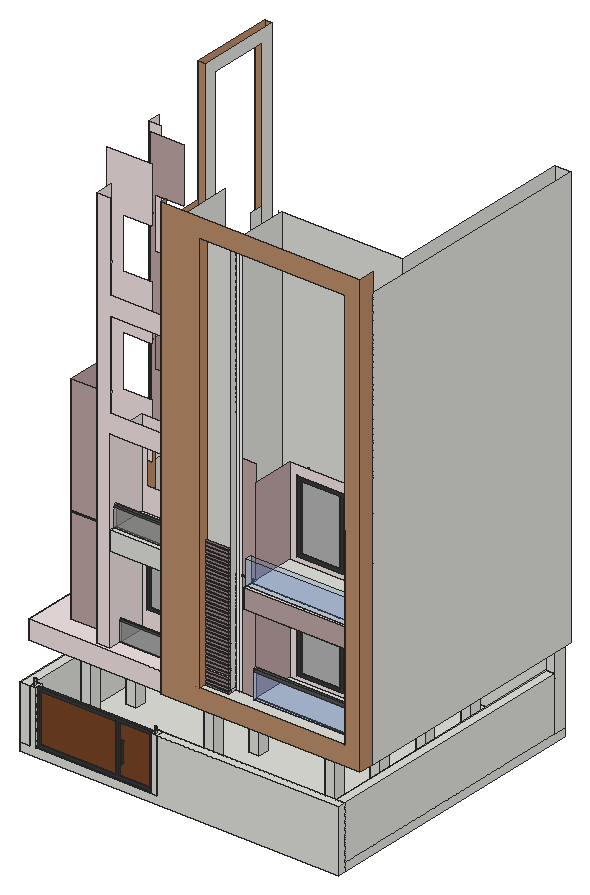
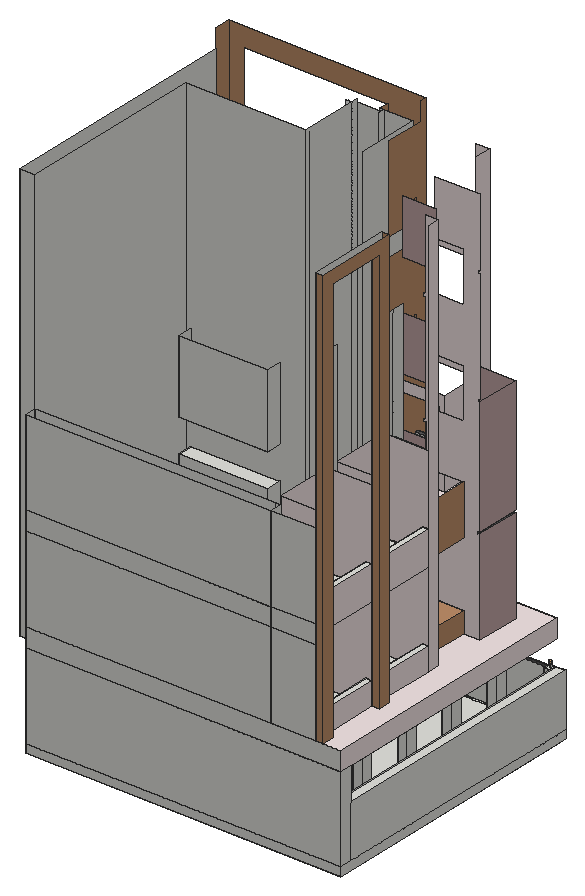
# SketchUp Ruby script. Lengths in inches.
U = 1.inch
M = Sketchup.active_model
def pt(a) = Geom::Point3d.new(a.map { |v| v * U })
def face(e, loops, mat)
  f = e.add_face(loops[0].map { |a| pt(a) })
  loops[1..].each { |l| e.add_face(l.map { |a| pt(a) }).erase! }
  f.material = f.back_material = mat if mat
  f
end
# faces: each face lists its corners as indices into pts; further lists are holes
def faces(e, pts, list, mat = nil) = list.each { |f| face(e, (f[0].is_a?(Array) ? f : [f]).map { |l| l.map { |i| pts[i] } }, mat) }
# xy, xz, yz: faces in a plane at the given z, y or x. An outline is a flat list of corners, or four numbers for a rectangle; further outlines are holes
def ring(l) = l.size == 4 ? [[l[0], l[1]], [l[2], l[1]], [l[2], l[3]], [l[0], l[3]]] : l.each_slice(2).to_a
def flat(e, list, mat, &to3) = list.each { |f| face(e, (f[0].is_a?(Array) ? f : [f]).map { |l| ring(l).map { |u, v| to3.(u, v) } }, mat) }
def xy(e, z, list, mat = nil) = flat(e, list, mat) { |x, y| [x, y, z] }
def xz(e, y, list, mat = nil) = flat(e, list, mat) { |x, z| [x, y, z] }
def yz(e, x, list, mat = nil) = flat(e, list, mat) { |y, z| [x, y, z] }
def lines(e, pts, list) = list.each { |a, b| e.add_line(pt(pts[a]), pt(pts[b])) }
# prism: a flat outline (further loops are holes) pulled along v
def prism(e, loops, v, mat = nil)
  f = face(e, loops, mat); d = Geom::Vector3d.new(v.map { |x| x * U })
  f.pushpull(f.normal.samedirection?(d) ? d.length : -d.length)
end
def box(e, o, s, mat = nil) = prism(e, [[o, [o[0] + s[0], o[1], o[2]], [o[0] + s[0], o[1] + s[1], o[2]], [o[0], o[1] + s[1], o[2]]]], [0, 0, s[2]], mat)
def at(x, y, z, deg = 0) = Geom::Transformation.translation(pt([x, y, z])) * Geom::Transformation.rotation(ORIGIN, Z_AXIS, deg.degrees)
def axes(o, x, y, z) = Geom::Transformation.new([*x, 0, *y, 0, *z, 0, *pt(o).to_a, 1])
def part(name) = M.definitions.add(name)
# library, detail: a bought-in or finely detailed component or shape, given as its bounding box
def library(name, o, s) = part(name).tap { |d| box(d.entities, o, s) }
def detail(e, o, s) = box(e.add_group.entities, o, s)
def put(e, d, t, mat = nil) = e.add_instance(d, t).tap { |i| i.material = mat if mat }
def group(e, t, mat = nil) = e.add_group.tap { |g| g.transformation = t; g.material = mat if mat }.entities
root = M.entities
M.materials.add("Generic\#1").color = [192, 166, 166]
M.materials.add("Generic\#2").color = [190, 142, 105]
M.materials.add("Generic\#3").color = [158, 131, 131]
M.materials.add("Generic\#4").color = [242, 228, 228]
M.materials.add("[Color M00]").color = [255, 255, 255]
M.materials.add("[Color M06]").color = [86, 86, 86]
M.materials.add("[Color M07]").color = [58, 58, 58]
M.materials.add("[Mirror 01]").color = [183, 183, 183]
M.materials.add("[Translucent Glass Blue]").color = [98, 147, 234]
M.materials["[Translucent Glass Blue]"].alpha = 0.21
M.materials.add("[Translucent Glass Gray]").color = [128, 128, 128]
M.materials["[Translucent Glass Gray]"].alpha = 0.5
M.materials.add("[Wood Veneer 01]").color = [120, 70, 37]
c1 = part("Group\#3")
xy(c1.entities,0,[[0,0,45.875,5.125]])
xz(c1.entities,0,[[0,0,45.875,4.1875]])
yz(c1.entities,45.875,[[0,0,5.125,4.1875]])
c2 = part("Group\#2")
xy(c2.entities,0,[[0,0,173,6]],"[Color M07]")
xy(c2.entities,7.67,[[90.33,0,165.33,3]],"[Color M06]")
xy(c2.entities,7.67,[[7.67,0,82.67,3]],"[Color M07]")
xy(c2.entities,134.58,[[7.67,0,82.67,3],[90.33,0,165.33,3]],"[Color M07]")
xy(c2.entities,142.25,[[0,0,173,6]],"[Color M07]")
xz(c2.entities,0,[[[0,0,173,142.25],[7.67,7.67,82.67,134.58],[90.33,7.67,165.33,134.58]]],"[Color M07]")
xz(c2.entities,3,[[7.67,7.67,82.67,134.58],[90.33,7.67,165.33,134.58]],"[Mirror 01]")
xz(c2.entities,6,[[0,0,173,142.25]],"[Mirror 01]")
yz(c2.entities,0,[[0,0,6,142.25]],"[Color M07]")
yz(c2.entities,7.67,[[0,7.67,3,134.58]],"[Color M07]")
yz(c2.entities,82.67,[[0,7.67,3,134.58]],"[Color M07]")
yz(c2.entities,90.33,[[0,7.67,3,134.58]],"[Color M07]")
yz(c2.entities,165.33,[[0,7.67,3,134.58]],"[Color M07]")
yz(c2.entities,173,[[0,0,6,142.25]],"[Color M07]")
c3 = part("Group\#1")
xy(c3.entities,0,[[0,0,90.75,6]],"[Color M07]")
xy(c3.entities,5.41,[[5.41,0,42.67,3],[48.08,0,85.34,3]],"[Color M07]")
xy(c3.entities,95.34,[[5.41,0,42.67,3],[48.08,0,85.34,3]],"[Color M07]")
xy(c3.entities,100.75,[[0,0,90.75,6]],"[Color M07]")
xz(c3.entities,0,[[[0,0,90.75,100.75],[48.08,5.41,85.34,95.34],[5.41,5.41,42.67,95.34]]],"[Color M07]")
xz(c3.entities,3,[[5.41,5.41,42.67,95.34],[48.08,5.41,85.34,95.34]],"[Mirror 01]")
xz(c3.entities,6,[[0,0,90.75,100.75]],"[Mirror 01]")
yz(c3.entities,0,[[0,0,6,100.75]],"[Color M07]")
yz(c3.entities,5.41,[[0,5.41,3,95.34]],"[Color M07]")
yz(c3.entities,42.67,[[0,5.41,3,95.34]],"[Color M07]")
yz(c3.entities,48.08,[[0,5.41,3,95.34]],"[Color M07]")
yz(c3.entities,85.34,[[0,5.41,3,95.34]],"[Color M07]")
yz(c3.entities,90.75,[[0,0,6,100.75]],"[Color M07]")
xy(root,-15.875,[[0,0,617.3125,15.0625],[0,15.0625,617.3125,549.6875]])
xy(root,0,[[0,0,18.4375,15.0625],[30.125,0,253,15.0625],[253,0,264.6875,15.0625],[0,15.0625,18.4375,525.6875],[[18.4375,15.0625,599.75,525.6875],[52.22,82.12,71.54,103.62],[52.22,191.41,71.54,212.91],[52.22,300.71,71.54,322.21],[52.22,410,71.54,431.5],[290.41,410,309.72,431.5],[290.41,300.71,309.72,322.21],[290.41,191.41,309.72,212.91],[290.41,82.12,309.72,103.62],[526.0625,410,545.375,431.5],[526.0625,300.71,545.375,322.21],[526.0625,191.41,545.375,212.91],[526.0625,82.12,545.375,103.62]],
  [599.75,15.0625,617.3125,525.6875],[52.22,82.12,71.54,103.62],[290.41,82.12,309.72,103.62],[526.0625,82.12,545.375,103.62],[52.22,191.41,71.54,212.91],
  [290.41,191.41,309.72,212.91],[526.0625,191.41,545.375,212.91],[52.22,300.71,71.54,322.21],[290.41,300.71,309.72,322.21],[526.0625,300.71,545.375,322.21],
  [52.22,410,71.54,431.5],[290.41,410,309.72,431.5],[526.0625,410,545.375,431.5],[0,525.6875,617.3125,549.6875]])
xy(root,104.18,[[0,0,18.4375,525.6875],[[18.4375,0,30.125,15.0625],[23.27,4.73,25.7,7.24]],[[253,0,264.6875,15.0625],[257.17,4.73,259.61,7.24]],[264.6875,0,617.3125,15.0625],[23.27,4.73,25.7,7.24],
  [257.17,4.73,259.61,7.24],[599.75,15.0625,617.3125,525.6875]])
xy(root,110.18,[[23.27,4.73,25.7,7.24],[257.17,4.73,259.61,7.24]])
xy(root,168,[[[261.3125,15.0625,261.3125,20.375,0,20.375,0,525.6875,647.125,525.6875,647.125,15.0625],[52.22,82.12,71.54,103.62],[52.22,191.41,71.54,212.91],[52.22,300.71,71.54,322.21],[52.22,410,71.54,431.5],[526.0625,82.12,545.375,103.62],[526.0625,191.41,545.375,212.91],[526.0625,300.71,545.375,322.21],[526.0625,410,545.375,431.5],[290.41,410,309.72,431.5],[290.41,300.71,309.72,322.21],[290.41,191.41,309.72,212.91],[290.41,82.12,309.72,103.62]],[0,525.6875,617.3125,549.6875]])
xy(root,204.5625,[[336,15.0625,617.3125,15.0625,617.3125,39,421.3125,39,421.3125,45.6875,381.875,45.6875,381.875,33.8125,336,33.8125],[271.74,33.8125,271.74,157.1,137.3125,157.1,137.3125,525.6875,617.3125,525.6875,617.3125,157.1,381.875,157.1,381.875,45.6875,328.375,45.6875,328.375,33.8125],[328.375,33.8125,381.875,45.6875],[421.3125,45.6875,617.3125,128.4375],[152.75,50.125,261.3125,53.5625],
  [80.75,147.9375,137.3125,225.85],[73.1875,225.85,137.3125,249.85],[49.25,249.85,137.3125,273.85],[61.25,273.85,137.3125,387.77],[34.875,387.77,49.25,411.77],
  [49.25,387.77,137.3125,411.77],[61.25,411.77,137.3125,525.6875],[34.875,525.6875,49.25,549.6875],[49.25,525.6875,137.3125,549.6875],[137.3125,525.6875,617.3125,549.6875]])
xy(root,204.5625,[[0,20.375,261.3125,20.375,261.3125,50.125,152.75,50.125,152.75,27.5625,126.1875,27.5625,126.1875,61.3125,49.25,61.3125,49.25,147.9375,80.75,147.9375,80.75,225.85,73.1875,225.85,73.1875,249.85,49.25,249.85,49.25,387.77,34.875,387.77,34.875,411.77,49.25,411.77,49.25,525.6875,34.875,525.6875,34.875,549.6875,0,549.6875]],"Generic\#4")
xy(root,204.5625,[[152.75,53.5625,261.3125,105]],"[Color M00]")
xy(root,209.0625,[[375.18,33.8125,381.875,157.1]])
xy(root,209.87,[[434.09,128.4375,607.09,187.0625]])
xy(root,240.21,[[162.625,105,253.375,171.75]])
xy(root,241.5,[[152.75,50.125,261.3125,53.5625]])
xy(root,245.0625,[[152.75,50.125,261.3125,53.5625]],"[Color M06]")
xy(root,245.625,[[80.75,147.9375,137.3125,225.85]],"Generic\#2")
xy(root,249.6875,[[49.25,273.85,61.25,387.77],[49.25,411.77,61.25,525.6875]])
xy(root,252.5625,[[421.3125,39,617.3125,45.6875]])
xy(root,258,[[421.3125,39,617.3125,45.6875]],"[Color M06]")
xy(root,340.96,[[162.625,105,253.375,171.75]])
xy(root,352.12,[[434.09,128.4375,607.09,187.0625]])
xy(root,372.5625,[[137.3125,525.6875,617.3125,549.6875]])
xy(root,372.5625,[[421.3125,15.0625,617.3125,128.4375],[80.75,147.9375,137.3125,225.85]],"Generic\#2")
xy(root,372.5625,[[152.75,27.5625,261.3125,105]],"Generic\#4")
xy(root,378.72,[[73.1875,225.85,77.875,249.85]],"[Color M06]")
xy(root,384.87,[[73.1875,225.85,77.875,249.85]],"[Color M06]")
xy(root,387.625,[[49.25,273.85,137.3125,387.77],[49.25,411.77,137.3125,525.6875]],"Generic\#4")
xy(root,390.07,[[49.25,61.3125,126.1875,66],[49.25,66,53.9375,147.9375]],"[Color M06]")
xy(root,394.07,[[49.25,61.3125,126.1875,66],[49.25,66,53.9375,147.9375]],"[Color M06]")
xy(root,406.125,[[392.6875,45.6875,421.3125,49.375]])
xy(root,409.125,[[421.3125,15.0625,617.3125,20.9],[421.3125,20.9,617.3125,32.9],[152.75,27.5625,261.3125,35.875],[421.3125,32.9,617.3125,128.4375],[152.75,35.875,261.3125,42.5625],
  [152.75,42.5625,261.3125,105],[392.6875,45.6875,421.3125,49.375],[61.25,273.85,137.3125,387.77],[61.25,411.77,137.3125,525.6875],[137.3125,525.6875,617.3125,549.6875]])
xy(root,417.43,[[434.09,128.4375,607.09,187.0625]])
xy(root,446.0625,[[152.75,35.875,261.3125,42.5625]])
xy(root,449.625,[[152.75,35.875,261.3125,42.5625]],"[Color M06]")
xy(root,454.25,[[49.25,273.85,61.25,387.77],[49.25,411.77,61.25,525.6875]])
xz(root,0,[[0,-15.875,617.3125,-15.875,617.3125,104.18,264.6875,104.18,264.6875,0,30.125,0,30.125,104.18,18.4375,104.18,18.4375,0,0,0],[0,0,18.4375,104.18],[253,0,264.6875,104.18]])
xz(root,4.73,[[23.27,104.18,25.7,110.18],[257.17,104.18,259.61,110.18]])
xz(root,7.24,[[23.27,104.18,25.7,110.18],[257.17,104.18,259.61,110.18]])
xz(root,15.0625,[[18.4375,0,30.125,104.18],[253,0,264.6875,104.18],[264.6875,0,599.75,104.18],[599.75,0,617.3125,104.18]])
xz(root,15.0625,[[421.3125,372.5625,617.3125,409.125]],"Generic\#1")
xz(root,15.0625,[[[261.3125,168,647.125,1022.8125],[336,204.5625,617.3125,986.25]]],"Generic\#2")
xz(root,20.375,[[0,168,261.3125,204.5625]],"Generic\#4")
xz(root,20.9,[[421.3125,409.125,617.3125,457.125]],"[Translucent Glass Blue]")
xz(root,27.5625,[[152.75,372.5625,261.3125,409.125]])
xz(root,27.5625,[[126.1875,204.5625,152.75,204.5625,152.75,577.125,261.3125,577.125,261.3125,613.6875,152.75,613.6875,152.75,781.6875,261.3125,781.6875,261.3125,818.25,152.75,818.25,152.75,986.25,126.1875,986.25]],"Generic\#4")
xz(root,32.9,[[421.3125,409.125,617.3125,457.125]],"[Translucent Glass Blue]")
xz(root,33.8125,[[271.74,204.5625,328.375,986.25],[328.375,204.5625,336,986.25],[336,204.5625,381.875,982.0625]])
xz(root,35.875,[[152.75,446.0625,261.3125,449.625]],"[Color M06]")
xz(root,35.875,[[152.75,409.125,261.3125,446.0625]],"[Translucent Glass Gray]")
xz(root,39,[[421.3125,252.5625,617.3125,258]],"[Color M06]")
xz(root,39,[[421.3125,204.5625,617.3125,252.5625]],"[Translucent Glass Blue]")
xz(root,42.5625,[[152.75,446.0625,261.3125,449.625]])
xz(root,42.5625,[[152.75,409.125,261.3125,446.0625]],"[Translucent Glass Gray]")
xz(root,45.6875,[[421.3125,252.5625,617.3125,258]])
xz(root,45.6875,[[392.6875,204.5625,421.3125,406.125],[392.6875,409.125,421.3125,610.6875]],"Generic\#1")
xz(root,45.6875,[[381.875,204.5625,392.6875,986.25]],"[Color M00]")
xz(root,45.6875,[[421.3125,204.5625,617.3125,252.5625]],"[Translucent Glass Blue]")
xz(root,49.375,[[392.6875,406.125,421.3125,409.125]],"[Color M06]")
xz(root,50.125,[[152.75,241.5,261.3125,245.0625]],"[Color M06]")
xz(root,50.125,[[152.75,204.5625,261.3125,241.5]],"[Translucent Glass Gray]")
xz(root,53.5625,[[152.75,241.5,261.3125,245.0625]])
xz(root,53.5625,[[152.75,204.5625,261.3125,241.5]],"[Translucent Glass Gray]")
xz(root,61.3125,[[49.25,204.5625,126.1875,390.07],[49.25,394.07,126.1875,621.63]],"Generic\#1")
xz(root,66,[[53.9375,390.07,126.1875,394.07]],"[Color M06]")
xz(root,82.12,[[52.22,0,71.54,168],[290.41,0,309.72,168],[526.0625,0,545.375,168]])
xz(root,103.62,[[52.22,0,71.54,168],[290.41,0,309.72,168],[526.0625,0,545.375,168]])
xz(root,105,[[[152.75,204.5625,261.3125,372.5625],[162.625,240.21,253.375,340.96]],[[152.75,409.125,261.3125,577.125],[162.5,455.21,253.25,555.96]]],"Generic\#4")
xz(root,128.4375,[[[421.3125,204.5625,617.3125,372.5625],[434.09,209.87,607.09,352.12]],[[421.3125,409.125,617.3125,577.125],[434.09,417.43,607.09,559.68]]],"Generic\#4")
xz(root,147.9375,[[80.75,204.5625,137.3125,245.625]])
xz(root,147.9375,[[49.25,204.5625,49.25,390.07,53.9375,390.07,53.9375,394.07,49.25,394.07,49.25,621.63,53.9375,621.63,53.9375,625.63,49.25,625.63,49.25,847.32,53.9375,847.32,53.9375,851.32,49.25,851.32,49.25,986.25,137.3125,986.25,137.3125,879.375,80.75,879.375,80.75,781.6875,137.3125,781.6875,137.3125,674.8125,80.75,674.8125,80.75,577.125,137.3125,577.125,137.3125,470.25,80.75,470.25,80.75,372.5625,137.3125,372.5625,137.3125,245.625,80.75,245.625,80.75,204.5625]],"Generic\#4")
xz(root,157.1,[[381.875,204.5625,617.3125,986.25]])
xz(root,171.75,[[162.625,240.21,253.375,340.96]])
xz(root,187.0625,[[434.09,209.87,607.09,352.12],[434.09,417.43,607.09,559.68]])
xz(root,191.41,[[52.22,0,71.54,168],[290.41,0,309.72,168],[526.0625,0,545.375,168]])
xz(root,212.91,[[52.22,0,71.54,168],[290.41,0,309.72,168],[526.0625,0,545.375,168]])
xz(root,225.85,[[80.75,204.5625,137.3125,245.625],[80.75,372.5625,137.3125,470.25]])
xz(root,225.85,[[73.1875,204.5625,80.75,204.5625,80.75,245.625,137.3125,245.625,137.3125,372.5625,80.75,372.5625,80.75,470.25,137.3125,470.25,137.3125,577.125,80.75,577.125,80.75,674.8125,137.3125,674.8125,137.3125,781.6875,80.75,781.6875,80.75,879.375,137.3125,879.375,137.3125,986.25,73.1875,986.25,73.1875,847.44,77.875,847.44,77.875,843.44,73.1875,843.44,73.1875,627.77,77.875,627.77,77.875,623.77,73.1875,623.77,73.1875,384.87,77.875,384.87,77.875,378.72,73.1875,378.72]],"Generic\#1")
xz(root,249.85,[[73.1875,204.5625,137.3125,372.5625],[73.1875,372.5625,137.3125,372.5625,137.3125,409.125,73.1875,409.125,73.1875,384.87,77.875,384.87,77.875,378.72,73.1875,378.72],[73.1875,409.125,137.3125,577.125]])
xz(root,249.85,[[49.25,204.5625,73.1875,204.5625,73.1875,378.72,77.875,378.72,77.875,384.87,73.1875,384.87,73.1875,623.77,77.875,623.77,77.875,627.77,73.1875,627.77,73.1875,843.44,77.875,843.44,77.875,847.44,73.1875,847.44,73.1875,986.25,49.25,986.25]],"Generic\#4")
xz(root,273.85,[[49.25,204.5625,61.25,249.6875],[49.25,387.625,49.25,454.25,61.25,454.25,61.25,409.125,137.3125,409.125,137.3125,387.625]])
xz(root,273.85,[[61.25,204.5625,61.25,249.6875,49.25,249.6875,49.25,387.625,137.3125,387.625,137.3125,204.5625],[61.25,409.125,61.25,454.25,49.25,454.25,49.25,592.1875,137.3125,592.1875,137.3125,409.125]],"Generic\#4")
xz(root,300.71,[[52.22,0,71.54,168],[290.41,0,309.72,168],[526.0625,0,545.375,168]])
xz(root,322.21,[[52.22,0,71.54,168],[290.41,0,309.72,168],[526.0625,0,545.375,168]])
xz(root,387.77,[[49.25,204.5625,61.25,249.6875],[49.25,387.625,137.3125,387.625,137.3125,409.125,61.25,409.125,61.25,454.25,49.25,454.25]])
xz(root,387.77,[[34.875,204.5625,49.25,1024.8125]],"Generic\#2")
xz(root,387.77,[[61.25,204.5625,137.3125,204.5625,137.3125,387.625,49.25,387.625,49.25,249.6875,61.25,249.6875],[61.25,409.125,137.3125,409.125,137.3125,592.1875,49.25,592.1875,49.25,454.25,61.25,454.25]],"Generic\#4")
xz(root,410,[[52.22,0,71.54,168],[290.41,0,309.72,168],[526.0625,0,545.375,168]])
xz(root,411.77,[[49.25,204.5625,61.25,249.6875],[49.25,387.625,49.25,454.25,61.25,454.25,61.25,409.125,137.3125,409.125,137.3125,387.625]])
xz(root,411.77,[[34.875,204.5625,49.25,1000.9375]],"Generic\#2")
xz(root,411.77,[[61.25,204.5625,61.25,249.6875,49.25,249.6875,49.25,387.625,137.3125,387.625,137.3125,204.5625],[61.25,409.125,61.25,454.25,49.25,454.25,49.25,592.1875,137.3125,592.1875,137.3125,409.125]],"Generic\#4")
xz(root,431.5,[[52.22,0,71.54,168],[290.41,0,309.72,168],[526.0625,0,545.375,168]])
xz(root,525.6875,[[0,0,18.4375,104.18],[18.4375,0,599.75,168],[599.75,0,617.3125,104.18],[0,104.18,18.4375,168],[599.75,104.18,617.3125,168],
  [617.3125,168,647.125,986.25],[49.25,204.5625,61.25,249.6875],[137.3125,204.5625,145.6875,372.5625],[145.6875,204.5625,617.3125,372.5625],[137.3125,372.5625,145.6875,409.125],
  [145.6875,372.5625,617.3125,409.125],[49.25,387.625,137.3125,387.625,137.3125,409.125,61.25,409.125,61.25,454.25,49.25,454.25],[137.3125,409.125,145.6875,577.125],[145.6875,409.125,617.3125,577.125]])
xz(root,525.6875,[[34.875,204.5625,49.25,1000.9375]],"Generic\#2")
xz(root,525.6875,[[61.25,204.5625,137.3125,204.5625,137.3125,387.625,49.25,387.625,49.25,249.6875,61.25,249.6875],[61.25,409.125,137.3125,409.125,137.3125,592.1875,49.25,592.1875,49.25,454.25,61.25,454.25]],"Generic\#4")
xz(root,549.6875,[[0,-15.875,617.3125,0],[0,0,617.3125,168],[0,168,617.3125,204.5625],[49.25,204.5625,137.3125,372.5625],[137.3125,204.5625,617.3125,372.5625],
  [49.25,372.5625,137.3125,409.125],[137.3125,372.5625,617.3125,409.125],[49.25,409.125,137.3125,577.125],[137.3125,409.125,617.3125,577.125]])
xz(root,549.6875,[[34.875,204.5625,49.25,1024.8125]],"Generic\#2")
yz(root,0,[[0,-15.875,549.6875,0],[0,0,525.6875,104.18],[525.6875,0,549.6875,168]])
yz(root,0,[[20.375,168,549.6875,204.5625]],"Generic\#4")
yz(root,18.4375,[[0,0,15.0625,104.18],[15.0625,0,525.6875,104.18]])
yz(root,23.27,[[4.73,104.18,7.24,110.18]])
yz(root,25.7,[[4.73,104.18,7.24,110.18]])
yz(root,30.125,[[0,0,15.0625,104.18]])
yz(root,34.875,[[387.77,204.5625,387.77,1024.8125,549.6875,1024.8125,549.6875,204.5625,525.6875,204.5625,525.6875,1000.9375,411.77,1000.9375,411.77,204.5625]],"Generic\#2")
yz(root,49.25,[[387.77,204.5625,411.77,204.5625,411.77,1000.9375,525.6875,1000.9375,525.6875,204.5625,549.6875,204.5625,549.6875,1024.8125,387.77,1024.8125]])
yz(root,49.25,[[61.3125,204.5625,147.9375,390.07],[61.3125,394.07,147.9375,621.63]],"Generic\#1")
yz(root,49.25,[[249.85,204.5625,273.85,986.25],[273.85,204.5625,387.77,249.6875],[411.77,204.5625,525.6875,249.6875],[273.85,387.625,387.77,454.25],[411.77,387.625,525.6875,454.25]],"Generic\#4")
yz(root,52.22,[[82.12,0,103.62,168],[191.41,0,212.91,168],[300.71,0,322.21,168],[410,0,431.5,168]])
yz(root,53.9375,[[66,390.07,147.9375,394.07]],"[Color M06]")
yz(root,61.25,[[273.85,204.5625,387.77,249.6875],[411.77,204.5625,525.6875,249.6875],[273.85,409.125,387.77,454.25],[411.77,409.125,525.6875,454.25]])
yz(root,71.54,[[82.12,0,103.62,168],[191.41,0,212.91,168],[300.71,0,322.21,168],[410,0,431.5,168]])
yz(root,73.1875,[[225.85,204.5625,249.85,378.72],[225.85,384.87,249.85,623.77]],"Generic\#1")
yz(root,77.875,[[225.85,378.72,249.85,384.87]],"[Color M06]")
yz(root,80.75,[[147.9375,204.5625,225.85,245.625],[147.9375,372.5625,225.85,470.25]],"Generic\#2")
yz(root,126.1875,[[27.5625,204.5625,27.5625,986.25,61.3125,986.25,61.3125,851.32,66,851.32,66,847.32,61.3125,847.32,61.3125,625.63,66,625.63,66,621.63,61.3125,621.63,61.3125,394.07,66,394.07,66,390.07,61.3125,390.07,61.3125,204.5625]],"Generic\#4")
yz(root,137.3125,[[147.9375,204.5625,157.1,245.625],[157.1,204.5625,225.85,245.625],[225.85,204.5625,249.85,796.75],[249.85,204.5625,273.85,796.75],[387.77,204.5625,411.77,796.75],
  [525.6875,204.5625,549.6875,372.5625],[157.1,372.5625,225.85,470.25],[525.6875,372.5625,549.6875,409.125],[273.85,387.625,387.77,409.125],[411.77,387.625,525.6875,409.125],
  [525.6875,409.125,549.6875,577.125]])
yz(root,137.3125,[[273.85,204.5625,387.77,387.625],[411.77,204.5625,525.6875,387.625],[147.9375,245.625,225.85,372.5625],[273.85,409.125,387.77,592.1875],[411.77,409.125,525.6875,592.1875]],"Generic\#4")
yz(root,152.75,[[50.125,204.5625,53.5625,241.5],[50.125,241.5,53.5625,245.0625],[27.5625,372.5625,45.6875,409.125],[35.875,409.125,42.5625,446.0625],[35.875,446.0625,42.5625,449.625]])
yz(root,152.75,[[27.5625,204.5625,50.125,204.5625,50.125,245.0625,53.5625,245.0625,53.5625,204.5625,105,204.5625,105,372.5625,27.5625,372.5625],[27.5625,409.125,35.875,409.125,35.875,449.625,42.5625,449.625,42.5625,409.125,105,409.125,105,577.125,27.5625,577.125]],"Generic\#4")
yz(root,162.625,[[105,240.21,171.75,340.96]])
yz(root,253,[[0,0,15.0625,104.18]])
yz(root,253.375,[[105,240.21,171.75,340.96]])
yz(root,257.17,[[4.73,104.18,7.24,110.18]])
yz(root,259.61,[[4.73,104.18,7.24,110.18]])
yz(root,261.3125,[[50.125,204.5625,53.5625,241.5],[50.125,241.5,53.5625,245.0625],[35.875,409.125,42.5625,446.0625],[35.875,446.0625,42.5625,449.625]])
yz(root,261.3125,[[15.0625,168,15.0625,1022.8125,27.5625,1022.8125,27.5625,986.25,105,986.25,105,818.25,45.6875,818.25,45.6875,858.75,36.375,858.75,36.375,818.25,27.5625,818.25,27.5625,781.6875,105,781.6875,105,613.6875,44.125,613.6875,44.125,654.1875,37.125,654.1875,37.125,613.6875,27.5625,613.6875,27.5625,577.125,105,577.125,105,409.125,42.5625,409.125,42.5625,449.625,35.875,449.625,35.875,409.125,27.5625,409.125,27.5625,372.5625,105,372.5625,105,204.5625,53.5625,204.5625,53.5625,245.0625,50.125,245.0625,50.125,204.5625,20.375,204.5625,20.375,168]],"Generic\#2")
yz(root,264.6875,[[0,0,15.0625,104.18]])
yz(root,271.74,[[33.8125,204.5625,157.1,986.25]])
yz(root,290.41,[[82.12,0,103.62,168],[191.41,0,212.91,168],[300.71,0,322.21,168],[410,0,431.5,168]])
yz(root,309.72,[[82.12,0,103.62,168],[191.41,0,212.91,168],[300.71,0,322.21,168],[410,0,431.5,168]])
yz(root,328.375,[[33.8125,204.5625,45.6875,986.25]])
yz(root,336,[[15.0625,204.5625,33.8125,204.5625,33.8125,982.0625,28.6875,982.0625,28.6875,986.25,15.0625,986.25]],"Generic\#2")
yz(root,381.875,[[33.8125,204.5625,45.6875,209.0625],[45.6875,204.5625,157.1,209.0625],[33.8125,209.0625,45.6875,986.25],[45.6875,209.0625,157.1,986.25]])
yz(root,392.6875,[[45.6875,406.125,49.375,409.125]])
yz(root,421.3125,[[39,204.5625,45.6875,252.5625],[39,252.5625,45.6875,258],[15.0625,372.5625,15.0625,409.125,49.375,409.125,49.375,406.125,45.6875,406.125,45.6875,372.5625],[20.9,409.125,32.9,457.125]])
yz(root,421.3125,[[45.6875,204.5625,128.4375,372.5625],[45.6875,409.125,128.4375,577.125]],"Generic\#1")
yz(root,434.09,[[128.4375,209.87,187.0625,352.12],[128.4375,417.43,187.0625,559.68]])
yz(root,526.0625,[[82.12,0,103.62,168],[191.41,0,212.91,168],[300.71,0,322.21,168],[410,0,431.5,168]])
yz(root,545.375,[[82.12,0,103.62,168],[191.41,0,212.91,168],[300.71,0,322.21,168],[410,0,431.5,168]])
yz(root,599.75,[[15.0625,0,525.6875,104.18]])
yz(root,607.09,[[128.4375,209.87,187.0625,352.12],[128.4375,417.43,187.0625,559.68]])
yz(root,617.3125,[[0,-15.875,15.0625,104.18],[15.0625,-15.875,549.6875,0],[15.0625,0,525.6875,104.18],[525.6875,0,549.6875,168],[525.6875,168,549.6875,204.5625],
  [157.1,204.5625,525.6875,986.25],[525.6875,204.5625,549.6875,372.5625],[39,252.5625,45.6875,258],[15.0625,372.5625,45.6875,409.125],[525.6875,372.5625,549.6875,409.125],
  [20.9,409.125,32.9,457.125],[525.6875,409.125,549.6875,577.125]])
yz(root,617.3125,[[15.0625,204.5625,15.0625,372.5625,128.4375,372.5625,128.4375,204.5625,45.6875,204.5625,45.6875,258,39,258,39,204.5625],[15.0625,409.125,15.0625,577.125,128.4375,577.125,128.4375,409.125,32.9,409.125,32.9,462.9375,20.9,462.9375,20.9,409.125]],"Generic\#2")
yz(root,647.125,[[45.6875,168,525.6875,986.25]])
yz(root,647.125,[[15.0625,168,45.6875,1022.8125]],"Generic\#2")
p = [[421.3125,45.6875,204.5625],[421.3125,45.6875,168],[328.375,45.6875,204.5625],[328.375,45.6875,168],[328.375,33.8125,204.5625],[328.375,15.0625,204.5625],
  [328.375,33.8125,168],[381.875,45.6875,204.5625],[381.875,45.6875,168],[392.6875,45.6875,204.5625],[392.6875,45.6875,168],[392.6875,41.875,986.25],
  [392.6875,41.875,168],[375.18,157.1,209.0625],[375.18,157.1,986.25],[381.875,33.8125,204.5625],[381.875,33.8125,168],[258.33,6.1,104.18],
  [258.33,6.1,110.18],[24.42,6.1,104.18],[24.42,6.1,110.18]]
lines(root,p,[[0,1],[2,3],[4,5],[4,6],[7,8],[9,10],[11,12],[13,14],[15,16],[17,18],[19,20]])
detail(root,[255.95,5.97,110.18],[5.11,0.13,5.44])
detail(root,[22.04,5.97,110.18],[5.11,0.13,5.44])
g1 = group(root,at(30.125,2.42,0))
xy(g1,0,[[0,1.58,222.875,7.58]],"[Color M07]")
xy(g1,5.38,[[5.38,1.58,152.18,4.58],[157.57,1.58,217.49,4.58]],"[Color M07]")
xy(g1,27.48,[[162.52,0,165.58,7.08]],"[Color M07]")
xy(g1,29.23,[[162.52,1.75,165.58,7.08]],"[Wood Veneer 01]")
xy(g1,66.46,[[162.52,1.75,165.58,4.58]],"[Color M07]")
xy(g1,68.21,[[162.52,0,165.58,4.58]],"[Color M07]")
xy(g1,98.8,[[5.38,1.58,152.18,4.58],[157.57,1.58,217.49,4.58]],"[Color M07]")
xy(g1,104.18,[[0,1.58,222.875,7.58]],"[Color M07]")
xz(g1,0,[[162.52,27.48,165.58,68.21]],"[Color M07]")
xz(g1,1.58,[[[0,0,222.875,104.18],[5.38,5.38,152.18,98.8],[157.57,5.38,217.49,98.8]]],"[Color M07]")
xz(g1,1.75,[[162.52,29.23,165.58,66.46]],"[Color M07]")
xz(g1,4.58,[[5.38,5.38,152.18,98.8],[[157.57,5.38,217.49,98.8],[162.52,66.46,165.58,68.21]],[162.52,66.46,165.58,68.21]],"[Wood Veneer 01]")
xz(g1,7.08,[[162.52,27.48,165.58,29.23]],"[Wood Veneer 01]")
xz(g1,7.58,[[0,0,222.875,104.18]])
yz(g1,0,[[1.58,0,7.58,104.18]],"[Color M07]")
yz(g1,5.38,[[1.58,5.38,4.58,98.8]],"[Color M07]")
yz(g1,152.18,[[1.58,5.38,4.58,98.8]],"[Color M07]")
yz(g1,157.57,[[1.58,5.38,4.58,98.8]],"[Color M07]")
yz(g1,162.52,[[0,27.48,0,68.21,4.58,68.21,4.58,66.46,1.75,66.46,1.75,29.23,7.08,29.23,7.08,27.48]],"[Color M07]")
yz(g1,165.58,[[0,27.48,7.08,27.48,7.08,29.23,1.75,29.23,1.75,66.46,4.58,66.46,4.58,68.21,0,68.21]],"[Color M07]")
yz(g1,217.49,[[1.58,5.38,4.58,98.8]],"[Color M07]")
yz(g1,222.875,[[1.58,0,7.58,104.18]],"[Color M07]")
p = [[163.93,0.58,28.07],[163.93,7.08,28.07],[163.93,4.58,67.63],[163.93,0.58,67.63]]
lines(g1,p,[[0,1],[2,3],[3,0]])
put(root,c1,at(336,28.6875,170.9375))
put(root,c1,at(336,28.6875,177.375))
put(root,c1,at(336,28.6875,183.8125))
put(root,c1,at(336,28.6875,190.25))
put(root,c1,at(336,28.6875,196.6875))
put(root,c1,at(336,28.6875,203.125),"Generic\#3")
put(root,c1,at(336,28.6875,209.5625),"Generic\#3")
put(root,c2,at(434.09,128.4375,209.87))
put(root,c1,at(336,28.6875,216),"Generic\#3")
put(root,c1,at(336,28.6875,222.4375),"Generic\#3")
put(root,c1,at(336,28.6875,228.875),"Generic\#3")
put(root,c1,at(336,28.6875,235.3125),"Generic\#3")
put(root,c3,at(162.625,105,240.21))
put(root,c1,at(336,28.6875,241.75),"Generic\#3")
put(root,c1,at(336,28.6875,248.1875),"Generic\#3")
put(root,c1,at(336,28.6875,254.625),"Generic\#3")
put(root,c1,at(336,28.6875,261.0625),"Generic\#3")
put(root,c1,at(336,28.6875,267.5),"Generic\#3")
put(root,c1,at(336,28.6875,273.9375),"Generic\#3")
put(root,c1,at(336,28.6875,280.375),"Generic\#3")
put(root,c1,at(336,28.6875,286.8125),"Generic\#3")
put(root,c1,at(336,28.6875,293.25),"Generic\#3")
put(root,c1,at(336,28.6875,299.6875),"Generic\#3")
put(root,c1,at(336,28.6875,306.125),"Generic\#3")
put(root,c1,at(336,28.6875,312.5625),"Generic\#3")
put(root,c1,at(336,28.6875,319),"Generic\#3")
put(root,c1,at(336,28.6875,325.4375),"Generic\#3")
put(root,c1,at(336,28.6875,331.875),"Generic\#3")
put(root,c1,at(336,28.6875,338.3125),"Generic\#3")
put(root,c1,at(336,28.6875,344.75),"Generic\#3")
put(root,c1,at(336,28.6875,351.1875),"Generic\#3")
put(root,c1,at(336,28.6875,357.625),"Generic\#3")
put(root,c1,at(336,28.6875,364.0625),"Generic\#3")
put(root,c1,at(336,28.6875,370.5),"Generic\#3")
put(root,c1,at(336,28.6875,376.9375),"Generic\#3")
put(root,c1,at(336,28.6875,383.375),"Generic\#3")
put(root,c1,at(336,28.6875,389.8125),"Generic\#3")
put(root,c1,at(336,28.6875,396.25),"Generic\#3")
put(root,c1,at(336,28.6875,402.6875),"Generic\#3")
put(root,c1,at(336,28.6875,409.125),"Generic\#3")
put(root,c1,at(336,28.6875,415.5625),"Generic\#3")
put(root,c2,at(434.09,128.4375,417.43))
put(root,c1,at(336,28.6875,422),"Generic\#3")
put(root,c1,at(336,28.6875,428.4375),"Generic\#3")
put(root,c1,at(336,28.6875,434.875),"Generic\#3")
put(root,c1,at(336,28.6875,441.3125),"Generic\#3")
put(root,c1,at(336,28.6875,447.75),"Generic\#3")
put(root,c1,at(336,28.6875,454.1875),"Generic\#3")
